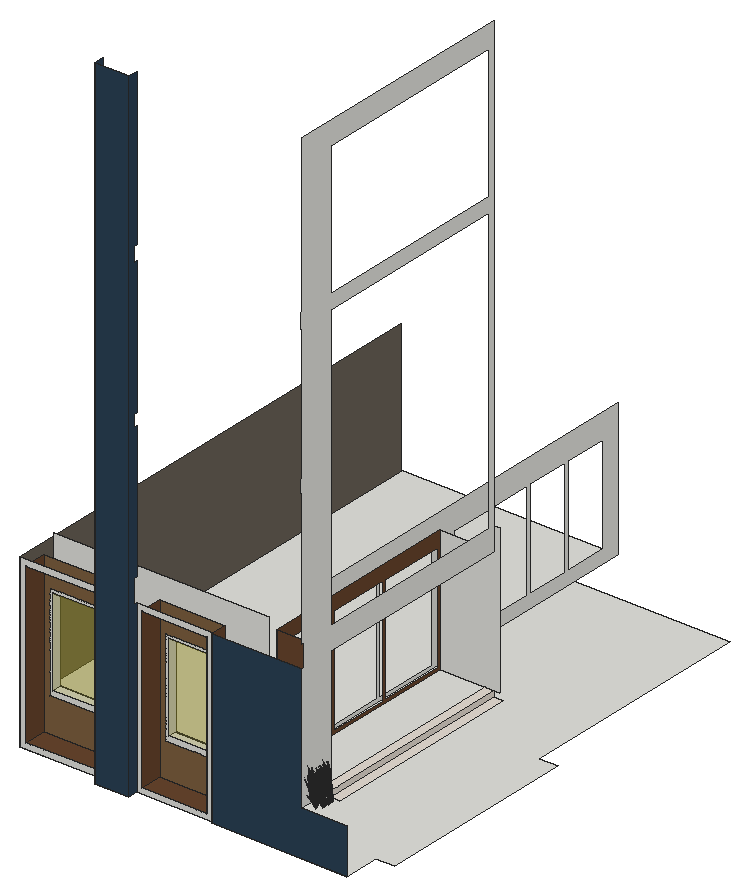
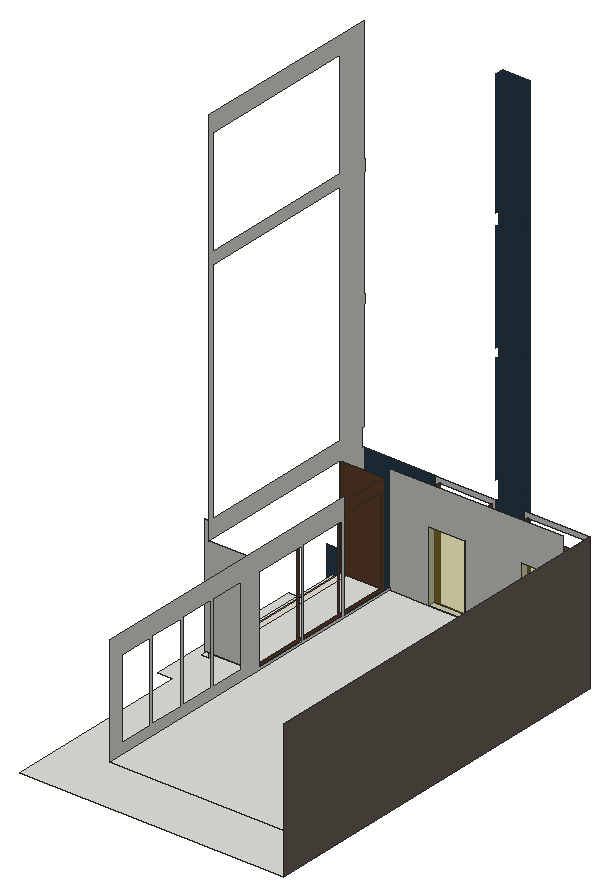
# SketchUp Ruby script. Lengths in inches.
U = 1.inch
M = Sketchup.active_model
def pt(a) = Geom::Point3d.new(a.map { |v| v * U })
def face(e, loops, mat)
  f = e.add_face(loops[0].map { |a| pt(a) })
  loops[1..].each { |l| e.add_face(l.map { |a| pt(a) }).erase! }
  f.material = f.back_material = mat if mat
  f
end
# faces: each face lists its corners as indices into pts; further lists are holes
def faces(e, pts, list, mat = nil) = list.each { |f| face(e, (f[0].is_a?(Array) ? f : [f]).map { |l| l.map { |i| pts[i] } }, mat) }
# xy, xz, yz: faces in a plane at the given z, y or x. An outline is a flat list of corners, or four numbers for a rectangle; further outlines are holes
def ring(l) = l.size == 4 ? [[l[0], l[1]], [l[2], l[1]], [l[2], l[3]], [l[0], l[3]]] : l.each_slice(2).to_a
def flat(e, list, mat, &to3) = list.each { |f| face(e, (f[0].is_a?(Array) ? f : [f]).map { |l| ring(l).map { |u, v| to3.(u, v) } }, mat) }
def xy(e, z, list, mat = nil) = flat(e, list, mat) { |x, y| [x, y, z] }
def xz(e, y, list, mat = nil) = flat(e, list, mat) { |x, z| [x, y, z] }
def yz(e, x, list, mat = nil) = flat(e, list, mat) { |y, z| [x, y, z] }
def lines(e, pts, list) = list.each { |a, b| e.add_line(pt(pts[a]), pt(pts[b])) }
# prism: a flat outline (further loops are holes) pulled along v
def prism(e, loops, v, mat = nil)
  f = face(e, loops, mat); d = Geom::Vector3d.new(v.map { |x| x * U })
  f.pushpull(f.normal.samedirection?(d) ? d.length : -d.length)
end
def box(e, o, s, mat = nil) = prism(e, [[o, [o[0] + s[0], o[1], o[2]], [o[0] + s[0], o[1] + s[1], o[2]], [o[0], o[1] + s[1], o[2]]]], [0, 0, s[2]], mat)
def at(x, y, z, deg = 0) = Geom::Transformation.translation(pt([x, y, z])) * Geom::Transformation.rotation(ORIGIN, Z_AXIS, deg.degrees)
def axes(o, x, y, z) = Geom::Transformation.new([*x, 0, *y, 0, *z, 0, *pt(o).to_a, 1])
def part(name) = M.definitions.add(name)
# library, detail: a bought-in or finely detailed component or shape, given as its bounding box
def library(name, o, s) = part(name).tap { |d| box(d.entities, o, s) }
def detail(e, o, s) = box(e.add_group.entities, o, s)
def put(e, d, t, mat = nil) = e.add_instance(d, t).tap { |i| i.material = mat if mat }
def group(e, t, mat = nil) = e.add_group.tap { |g| g.transformation = t; g.material = mat if mat }.entities
root = M.entities
M.materials.add("Carpet_04_1K").color = [43, 65, 85]
M.materials.add("Glass_Basic_1").color = [186, 174, 38]
M.materials["Glass_Basic_1"].alpha = 0.25
M.materials.add("LightPink_Translucent").color = [144, 107, 117]
M.materials["LightPink_Translucent"].alpha = 0.75
M.materials.add("Marble_01_1K").color = [230, 221, 211]
M.materials.add("Plaster_04_1K").color = [106, 98, 87]
M.materials.add("Plywood_01_1K").color = [125, 96, 64]
M.materials.add("Wood_Veneer_15_1K").color = [103, 69, 45]
c1 = part("blade")
p = [[2.15,0.21,22],[0,0.17,0],[0.09,0.45,0],[2.18,0.31,22],[2.29,0.31,22],[0.38,0.45,0],
  [2.48,0.24,33],[2.49,0.24,33],[2.48,0.22,33]]
faces(c1.entities,p,[[0,1,2,3],[4,5,2,3],[6,3,4,7],[8,0,3,6]])
c2 = part("seeds")
p = [[0.3,-0.1,1.38],[-0.01,-0.03,1.59],[-0.01,-0.03,0.03],[0.14,-0.07,-0.07],[0.29,-0.03,3],[0.15,0.01,3.11]]
faces(c2.entities,p,[[0,1,2,3],[1,0,4,5]],"LightPink_Translucent")
c3 = part("blade with seeds")
put(c3.entities,c1,at(0,0,0))
put(c3.entities,c2,axes([2.4,0.25,30.99],[1.5799,-0.05474,1.17369],[-0.12525,1.92788,0.29478],[-0.07173,-0.02425,1.56792]))
xy(root,0,[[91,0,91,10,4,10,4,514,352,514,352,262,372,262,372,46,352,46,352,8,208,8,208,10,127,10,127,0]])
xy(root,6,[[10,10,85,34],[133,10,202,34]],"Wood_Veneer_15_1K")
xy(root,42,[[304,46,314,262]],"Marble_01_1K")
xy(root,48,[[19,34,67,43],[142,34,190,43],[13,43,241,505],[247,46,295,262]])
xy(root,48,[[295,46,304,262]],"Marble_01_1K")
xz(root,0,[[91,0,127,684]],"Carpet_04_1K")
xz(root,8,[[208,0,352,0,352,48,304,48,304,180,208,180]],"Carpet_04_1K")
xz(root,10,[[[4,0,91,180],[10,6,85,174]],[[127,0,208,180],[133,6,202,174]]])
xz(root,34,[[[16,42,70,144],[19,48,67,141]],[[139,42,193,144],[142,48,190,141]]])
xz(root,34,[[19,48,67,141],[142,48,190,141]],"Glass_Basic_1")
xz(root,34,[[[10,6,85,174],[16,42,70,144]],[[133,6,202,174],[139,42,193,144]]],"Plywood_01_1K")
xz(root,43,[[13,48,13,192,241,192,241,48,190,48,190,141,142,141,142,48,67,48,67,141,19,141,19,48]])
xz(root,43,[[19,48,67,141],[142,48,190,141]],"Glass_Basic_1")
xz(root,46,[[247,48,304,180]],"Wood_Veneer_15_1K")
xz(root,262,[[247,48,310,48,310,204,304,204,304,180,247,180]])
yz(root,4,[[10,0,514,180]],"Plaster_04_1K")
yz(root,10,[[10,6,34,174]],"Wood_Veneer_15_1K")
yz(root,19,[[34,48,43,141]])
yz(root,67,[[34,48,43,141]])
yz(root,85,[[10,6,34,174]],"Wood_Veneer_15_1K")
yz(root,91,[[0,0,0,684,10,684,10,519,6,519,6,504,10,504,10,360,6,360,6,348,10,348,10,204,6,204,6,180,10,180,10,0]],"Carpet_04_1K")
yz(root,127,[[0,0,10,0,10,180,6,180,6,204,10,204,10,348,6,348,6,360,10,360,10,504,6,504,6,519,10,519,10,684,0,684]],"Carpet_04_1K")
yz(root,133,[[10,6,34,174]],"Wood_Veneer_15_1K")
yz(root,142,[[34,48,43,141]])
yz(root,190,[[34,48,43,141]])
yz(root,202,[[10,6,34,174]],"Wood_Veneer_15_1K")
yz(root,208,[[8,0,10,180]],"Carpet_04_1K")
yz(root,241,[[[43,48,43,51,119,51,119,192,505,192,505,48],[189,51,259,165],[122,51,186,165],[288,62,334.25,166],[338.25,62,384.5,166],[388.5,62,434.75,166],[438.75,62,485,166]]])
yz(root,247,[[[46,48,262,180],[189,51,259,165],[49,51,119,165],[122,51,186,165]]],"Wood_Veneer_15_1K")
yz(root,304,[[[8,48,46,48,46,180,262,180,262,684,8,684,8,519,6,519,6,504,8,504,8,360,6,360,6,348,8,348,8,204,10,204,10,180,8,180],[46,204,46,504,256,504,256,519,46,519,46,660,256,660,256,204]]])
yz(root,304,[[46,42,262,48]],"Marble_01_1K")
put(root,c3,axes([311.91,16.14,48.62],[0.20943,-0.00885,1.51428],[-0.13893,0.38357,0.12244],[-0.29846,-0.02372,0.64734]))
put(root,c3,axes([312.22,36.27,45.43],[0.20943,-0.00885,1.51428],[-0.13893,0.38357,0.12244],[-0.29846,-0.02372,0.64734]))
put(root,c3,axes([312,16.82,48.62],[0.17519,-0.08265,1.51428],[0.14749,0.38193,0.12244],[-0.27504,0.08632,0.64734]))
put(root,c3,axes([312.44,30.6,45.43],[0.20943,-0.00885,1.51428],[-0.13893,0.38357,0.12244],[-0.29846,-0.02372,0.64734]))
put(root,c3,axes([312.45,25.09,45.43],[0.20943,-0.00885,1.51428],[-0.13893,0.38357,0.12244],[-0.29846,-0.02372,0.64734]))
put(root,c3,axes([311.45,17.47,47.49],[0.17547,0.03208,1.26356],[0.1131,0.32764,-0.27174],[-0.23835,0.06133,0.54024]))
put(root,c3,axes([313,16.42,48.15],[0.14352,-0.05653,1.56454],[0.04949,0.39467,0.12244],[-0.31087,0.05237,0.55918]))
put(root,c3,axes([312.31,36.94,45.43],[0.17519,-0.08265,1.51428],[0.14749,0.38193,0.12244],[-0.27504,0.08632,0.64734]))
put(root,c3,axes([311.76,37.59,44.29],[0.17547,0.03208,1.26356],[0.1131,0.32764,-0.27174],[-0.23835,0.06133,0.54024]))
put(root,c3,axes([312.53,31.27,45.43],[0.17519,-0.08265,1.51428],[0.14749,0.38193,0.12244],[-0.27504,0.08632,0.64734]))
put(root,c3,axes([312.54,25.77,45.43],[0.17519,-0.08265,1.51428],[0.14749,0.38193,0.12244],[-0.27504,0.08632,0.64734]))
put(root,c3,axes([313.3125,36.55,44.95],[0.14352,-0.05653,1.56454],[0.04949,0.39467,0.12244],[-0.31087,0.05237,0.55918]))
put(root,c3,axes([311.46,16.68,49.36],[-0.08245,0.05073,1.54581],[0.00701,0.37067,-0.24447],[-0.18899,0.0482,0.12397]))
put(root,c3,axes([312.53,15.79,49.6],[-0.50473,-0.00941,-0.62776],[0.0339,-0.39618,0.07576],[-0.21383,-0.04181,0.88802]))
put(root,c3,axes([311.98,31.92,44.29],[0.17547,0.03208,1.26356],[0.1131,0.32764,-0.27174],[-0.23835,0.06133,0.54024]))
put(root,c3,axes([312,26.42,44.29],[0.17547,0.03208,1.26356],[0.1131,0.32764,-0.27174],[-0.23835,0.06133,0.54024]))
put(root,c3,axes([312.13,15.88,47.49],[0.09858,0.10879,1.26356],[-0.22716,0.29571,-0.27174],[-0.23325,-0.07068,0.54024]))
put(root,c3,axes([311.72,16.47,49.2],[-0.41962,-0.10901,-0.31292],[0.12239,-0.31802,0.40398],[-0.16894,0.02916,0.77298]))
put(root,c3,axes([312.3,15.53,48.62],[0.18755,0.06732,1.51428],[-0.38813,0.28243,0.12244],[-0.24191,-0.12741,0.64734]))
put(root,c3,axes([313.54,30.875,44.95],[0.14352,-0.05653,1.56454],[0.04949,0.39467,0.12244],[-0.31087,0.05237,0.55918]))
put(root,c3,axes([313.55,25.37,44.95],[0.14352,-0.05653,1.56454],[0.04949,0.39467,0.12244],[-0.31087,0.05237,0.55918]))
put(root,c3,axes([311.77,36.81,46.17],[-0.08245,0.05073,1.54581],[0.00701,0.37067,-0.24447],[-0.18899,0.0482,0.12397]))
put(root,c3,axes([312.85,35.91,46.4],[-0.50473,-0.00941,-0.62776],[0.0339,-0.39618,0.07576],[-0.21383,-0.04181,0.88802]))
put(root,c3,axes([310.54,17.06,49.36],[0.06444,0.01048,1.56736],[0.19934,0.34525,-0.1481],[-0.13191,0.09062,0.27737]))
put(root,c3,axes([312.01,16.64,49.33],[-0.13679,0.35544,-0.45151],[-0.46898,-0.12183,-0.34973],[-0.18882,0.03259,0.86392]))
put(root,c3,axes([312.4375,36.01,44.29],[0.09858,0.10879,1.26356],[-0.22716,0.29571,-0.27174],[-0.23325,-0.07068,0.54024]))
put(root,c3,axes([312.03,36.6,46],[-0.41962,-0.10901,-0.31292],[0.12239,-0.31802,0.40398],[-0.16894,0.02916,0.77298]))
put(root,c3,axes([312.37,15.87,49.33],[-0.36663,0.25884,-0.45151],[-0.32109,-0.27343,-0.34973],[-0.18628,-0.03938,0.86392]))
put(root,c3,axes([311.78,16.61,46.52],[0.0128,0.06158,1.55816],[-0.25814,0.3216,-0.23804],[-0.18336,-0.01621,0.26541]))
put(root,c3,axes([312.62,35.65,45.43],[0.18755,0.06732,1.51428],[-0.38813,0.28243,0.12244],[-0.24191,-0.12741,0.64734]))
put(root,c3,axes([311.99,31.14,46.17],[-0.08245,0.05073,1.54581],[0.00701,0.37067,-0.24447],[-0.18899,0.0482,0.12397]))
put(root,c3,axes([312.01,25.63,46.17],[-0.08245,0.05073,1.54581],[0.00701,0.37067,-0.24447],[-0.18899,0.0482,0.12397]))
put(root,c3,axes([313.07,30.24,46.4],[-0.50473,-0.00941,-0.62776],[0.0339,-0.39618,0.07576],[-0.21383,-0.04181,0.88802]))
put(root,c3,axes([313.08,24.74,46.4],[-0.50473,-0.00941,-0.62776],[0.0339,-0.39618,0.07576],[-0.21383,-0.04181,0.88802]))
put(root,c3,axes([312.66,30.34,44.29],[0.09858,0.10879,1.26356],[-0.22716,0.29571,-0.27174],[-0.23325,-0.07068,0.54024]))
put(root,c3,axes([312.67,24.83,44.29],[0.09858,0.10879,1.26356],[-0.22716,0.29571,-0.27174],[-0.23325,-0.07068,0.54024]))
put(root,c3,axes([311.85,15.14,49.36],[0.03743,0.039,1.56736],[-0.18045,0.35054,-0.1481],[-0.18276,0.00254,0.27737]))
put(root,c3,axes([310.85,37.18,46.16],[0.06444,0.01048,1.56736],[0.19934,0.34525,-0.1481],[-0.13191,0.09062,0.27737]))
put(root,c3,axes([312.32,36.76,46.14],[-0.13679,0.35544,-0.45151],[-0.46898,-0.12183,-0.34973],[-0.18882,0.03259,0.86392]))
put(root,c3,axes([312.26,30.93,46],[-0.41962,-0.10901,-0.31292],[0.12239,-0.31802,0.40398],[-0.16894,0.02916,0.77298]))
put(root,c3,axes([312.27,25.42,46],[-0.41962,-0.10901,-0.31292],[0.12239,-0.31802,0.40398],[-0.16894,0.02916,0.77298]))
put(root,c3,axes([312.84,29.98,45.43],[0.18755,0.06732,1.51428],[-0.38813,0.28243,0.12244],[-0.24191,-0.12741,0.64734]))
put(root,c3,axes([311.08,18.16,47.64],[0.21042,-0.1771,1.01491],[0.08303,0.28036,0.74569],[-0.15207,0.0502,0.22354]))
put(root,c3,axes([312.85,24.48,45.43],[0.18755,0.06732,1.51428],[-0.38813,0.28243,0.12244],[-0.24191,-0.12741,0.64734]))
put(root,c3,axes([312.27,14.91,49.36],[-0.10864,-0.00276,1.54581],[-0.34587,0.27582,-0.24447],[-0.18454,-0.05636,0.12397]))
put(root,c3,axes([312.68,35.99,46.14],[-0.36663,0.25884,-0.45151],[-0.32109,-0.27343,-0.34973],[-0.18628,-0.03938,0.86392]))
put(root,c3,axes([312.09,36.74,43.32],[0.0128,0.06158,1.55816],[-0.25814,0.3216,-0.23804],[-0.18336,-0.01621,0.26541]))
put(root,c3,axes([311.82,16.43,49.38],[0.14265,-0.35629,0.42415],[0.46898,0.12183,0.34973],[-0.18443,0.02141,0.87768]))
put(root,c3,axes([311.99,16.33,49.64],[0.25405,0.35383,-0.10745],[-0.45089,0.17388,-0.59638],[-0.19001,0.04668,0.90619]))
put(root,c3,axes([311.08,31.51,46.16],[0.06444,0.01048,1.56736],[0.19934,0.34525,-0.1481],[-0.13191,0.09062,0.27737]))
put(root,c3,axes([312.55,31.09,46.14],[-0.13679,0.35544,-0.45151],[-0.46898,-0.12183,-0.34973],[-0.18882,0.03259,0.86392]))
put(root,c3,axes([311.09,26.01,46.16],[0.06444,0.01048,1.56736],[0.19934,0.34525,-0.1481],[-0.13191,0.09062,0.27737]))
put(root,c3,axes([312.56,25.59,46.14],[-0.13679,0.35544,-0.45151],[-0.46898,-0.12183,-0.34973],[-0.18882,0.03259,0.86392]))
put(root,c3,axes([312.56,15.6,49.64],[-0.02704,0.39739,-0.10745],[-0.51189,-0.01086,-0.59638],[-0.19715,-0.0276,0.90619]))
put(root,c3,axes([312.23,15.625,49.2],[-0.28729,-0.24465,-0.31292],[0.32804,-0.23159,0.40398],[-0.16667,-0.03524,0.77298]))
put(root,c3,axes([312.16,35.27,46.16],[0.03743,0.039,1.56736],[-0.18045,0.35054,-0.1481],[-0.18276,0.00254,0.27737]))
put(root,c3,axes([311.79,16.34,49.375],[-0.18545,-0.26643,0.05682],[0.33817,-0.13041,0.44729],[-0.14907,0.02573,0.68204]))
put(root,c3,axes([312.64,17.08,48.62],[0.12611,-0.12006,1.51428],[0.31843,0.32408,0.12244],[-0.2184,0.14759,0.64734]))
put(root,c3,axes([312.9,30.32,46.14],[-0.36663,0.25884,-0.45151],[-0.32109,-0.27343,-0.34973],[-0.18628,-0.03938,0.86392]))
put(root,c3,axes([311.88,17.39,49.2],[-0.43951,0.05584,-0.31292],[-0.11606,-0.31924,0.40398],[-0.12595,0.08575,0.77298]))
put(root,c3,axes([312.91,24.82,46.14],[-0.36663,0.25884,-0.45151],[-0.32109,-0.27343,-0.34973],[-0.18628,-0.03938,0.86392]))
put(root,c3,axes([312.31,31.07,43.32],[0.0128,0.06158,1.55816],[-0.25814,0.3216,-0.23804],[-0.18336,-0.01621,0.26541]))
put(root,c3,axes([311.39,38.28,44.44],[0.21042,-0.1771,1.01491],[0.08303,0.28036,0.74569],[-0.15207,0.0502,0.22354]))
put(root,c3,axes([312.32,25.5625,43.32],[0.0128,0.06158,1.55816],[-0.25814,0.3216,-0.23804],[-0.18336,-0.01621,0.26541]))
put(root,c3,axes([312.58,35.03,46.17],[-0.10864,-0.00276,1.54581],[-0.34587,0.27582,-0.24447],[-0.18454,-0.05636,0.12397]))
put(root,c3,axes([311.64,18.34,46.52],[0.06773,0.03904,1.55816],[0.11484,0.36171,-0.23804],[-0.15011,0.07713,0.26541]))
put(root,c3,axes([311.54,16.21,47.64],[0.32236,-0.02796,1.01491],[-0.20448,0.24636,0.74569],[-0.1593,-0.03696,0.22354]))
put(root,c3,axes([312.38,29.6,46.16],[0.03743,0.039,1.56736],[-0.18045,0.35054,-0.1481],[-0.18276,0.00254,0.27737]))
put(root,c3,axes([312.13,36.56,46.18],[0.14265,-0.35629,0.42415],[0.46898,0.12183,0.34973],[-0.18443,0.02141,0.87768]))
put(root,c3,axes([312.4,24.09,46.16],[0.03743,0.039,1.56736],[-0.18045,0.35054,-0.1481],[-0.18276,0.00254,0.27737]))
put(root,c3,axes([312.3,36.46,46.45],[0.25405,0.35383,-0.10745],[-0.45089,0.17388,-0.59638],[-0.19001,0.04668,0.90619]))
put(root,c3,axes([312.87,35.72,46.45],[-0.02704,0.39739,-0.10745],[-0.51189,-0.01086,-0.59638],[-0.19715,-0.0276,0.90619]))
put(root,c3,axes([312.54,35.75,46],[-0.28729,-0.24465,-0.31292],[0.32804,-0.23159,0.40398],[-0.16667,-0.03524,0.77298]))
put(root,c3,axes([311.62,32.61,44.44],[0.21042,-0.1771,1.01491],[0.08303,0.28036,0.74569],[-0.15207,0.0502,0.22354]))
put(root,c3,axes([311.63,27.11,44.44],[0.21042,-0.1771,1.01491],[0.08303,0.28036,0.74569],[-0.15207,0.0502,0.22354]))
put(root,c3,axes([312.1,36.46,46.18],[-0.18545,-0.26643,0.05682],[0.33817,-0.13041,0.44729],[-0.14907,0.02573,0.68204]))
put(root,c3,axes([312.8,29.36,46.17],[-0.10864,-0.00276,1.54581],[-0.34587,0.27582,-0.24447],[-0.18454,-0.05636,0.12397]))
put(root,c3,axes([311.93,17.32,49.38],[-0.12522,-0.35963,0.42415],[0.49122,-0.06241,0.34973],[-0.14477,0.08458,0.87768]))
put(root,c3,axes([312.95,37.2,45.43],[0.12611,-0.12006,1.51428],[0.31843,0.32408,0.12244],[-0.2184,0.14759,0.64734]))
put(root,c3,axes([312.8125,23.86,46.17],[-0.10864,-0.00276,1.54581],[-0.34587,0.27582,-0.24447],[-0.18454,-0.05636,0.12397]))
put(root,c3,axes([312.1875,37.52,46],[-0.43951,0.05584,-0.31292],[-0.11606,-0.31924,0.40398],[-0.12595,0.08575,0.77298]))
put(root,c3,axes([312.36,30.89,46.18],[0.14265,-0.35629,0.42415],[0.46898,0.12183,0.34973],[-0.18443,0.02141,0.87768]))
put(root,c3,axes([312.1875,15.53,49.7],[0.41698,-0.28837,0.47505],[0.35962,0.30624,0.3917],[-0.19563,-0.05319,0.983]))
put(root,c3,axes([312.37,25.38,46.18],[0.14265,-0.35629,0.42415],[0.46898,0.12183,0.34973],[-0.18443,0.02141,0.87768]))
put(root,c3,axes([311.95,38.46,43.32],[0.06773,0.03904,1.55816],[0.11484,0.36171,-0.23804],[-0.15011,0.07713,0.26541]))
put(root,c3,axes([312.52,30.78,46.45],[0.25405,0.35383,-0.10745],[-0.45089,0.17388,-0.59638],[-0.19001,0.04668,0.90619]))
put(root,c3,axes([311.84,17.25,49.375],[-0.34663,-0.16434,0.05682],[0.20181,-0.23402,0.44729],[-0.11113,0.07566,0.68204]))
put(root,c3,axes([312.54,25.28,46.45],[0.25405,0.35383,-0.10745],[-0.45089,0.17388,-0.59638],[-0.19001,0.04668,0.90619]))
put(root,c3,axes([313.09,30.05,46.45],[-0.02704,0.39739,-0.10745],[-0.51189,-0.01086,-0.59638],[-0.19715,-0.0276,0.90619]))
put(root,c3,axes([311.85,36.34,44.44],[0.32236,-0.02796,1.01491],[-0.20448,0.24636,0.74569],[-0.1593,-0.03696,0.22354]))
put(root,c3,axes([313.11,24.55,46.45],[-0.02704,0.39739,-0.10745],[-0.51189,-0.01086,-0.59638],[-0.19715,-0.0276,0.90619]))
put(root,c3,axes([312.76,30.08,46],[-0.28729,-0.24465,-0.31292],[0.32804,-0.23159,0.40398],[-0.16667,-0.03524,0.77298]))
put(root,c3,axes([312.78,24.57,46],[-0.28729,-0.24465,-0.31292],[0.32804,-0.23159,0.40398],[-0.16667,-0.03524,0.77298]))
put(root,c3,axes([312.32,30.79,46.18],[-0.18545,-0.26643,0.05682],[0.33817,-0.13041,0.44729],[-0.14907,0.02573,0.68204]))
put(root,c3,axes([312.33,25.29,46.18],[-0.18545,-0.26643,0.05682],[0.33817,-0.13041,0.44729],[-0.14907,0.02573,0.68204]))
put(root,c3,axes([313.17,31.53,45.43],[0.12611,-0.12006,1.51428],[0.31843,0.32408,0.12244],[-0.2184,0.14759,0.64734]))
put(root,c3,axes([312.41,31.84,46],[-0.43951,0.05584,-0.31292],[-0.11606,-0.31924,0.40398],[-0.12595,0.08575,0.77298]))
put(root,c3,axes([313.18,26.03,45.43],[0.12611,-0.12006,1.51428],[0.31843,0.32408,0.12244],[-0.2184,0.14759,0.64734]))
put(root,c3,axes([312.42,26.34,46],[-0.43951,0.05584,-0.31292],[-0.11606,-0.31924,0.40398],[-0.12595,0.08575,0.77298]))
put(root,c3,axes([312.54,17.37,48.62],[0.09401,-0.13431,1.51428],[0.3944,0.27795,0.12244],[-0.17792,0.17323,0.64734]))
put(root,c3,axes([312.25,37.45,46.18],[-0.12522,-0.35963,0.42415],[0.49122,-0.06241,0.34973],[-0.14477,0.08458,0.87768]))
put(root,c3,axes([312.17,32.79,43.32],[0.06773,0.03904,1.55816],[0.11484,0.36171,-0.23804],[-0.15011,0.07713,0.26541]))
put(root,c3,axes([312.18,27.29,43.32],[0.06773,0.03904,1.55816],[0.11484,0.36171,-0.23804],[-0.15011,0.07713,0.26541]))
put(root,c3,axes([312.07,30.66,44.44],[0.32236,-0.02796,1.01491],[-0.20448,0.24636,0.74569],[-0.1593,-0.03696,0.22354]))
put(root,c3,axes([312.09,25.16,44.44],[0.32236,-0.02796,1.01491],[-0.20448,0.24636,0.74569],[-0.1593,-0.03696,0.22354]))
put(root,c3,axes([312.5,35.66,46.5],[0.41698,-0.28837,0.47505],[0.35962,0.30624,0.3917],[-0.19563,-0.05319,0.983]))
put(root,c3,axes([312.15,37.375,46.18],[-0.34663,-0.16434,0.05682],[0.20181,-0.23402,0.44729],[-0.11113,0.07566,0.68204]))
put(root,c3,axes([312.17,16.4375,49.66],[0.41962,0.10901,0.31292],[-0.12239,0.31802,-0.40398],[-0.16894,0.02916,0.77298]))
